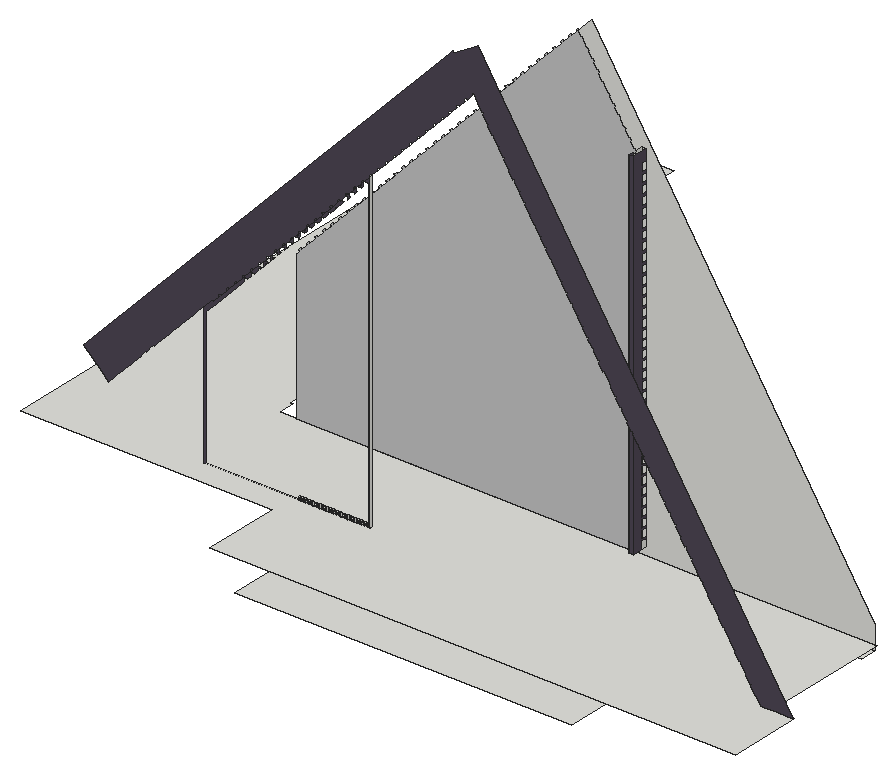
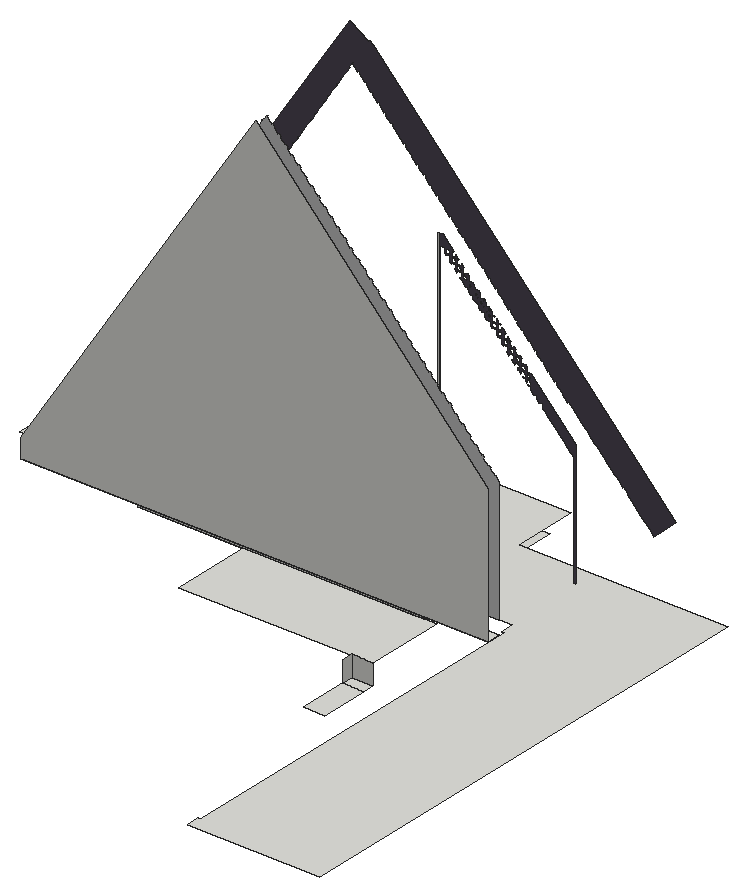
# SketchUp Ruby script. Lengths in inches.
U = 1.inch
M = Sketchup.active_model
def pt(a) = Geom::Point3d.new(a.map { |v| v * U })
def face(e, loops, mat)
  f = e.add_face(loops[0].map { |a| pt(a) })
  loops[1..].each { |l| e.add_face(l.map { |a| pt(a) }).erase! }
  f.material = f.back_material = mat if mat
  f
end
# faces: each face lists its corners as indices into pts; further lists are holes
def faces(e, pts, list, mat = nil) = list.each { |f| face(e, (f[0].is_a?(Array) ? f : [f]).map { |l| l.map { |i| pts[i] } }, mat) }
# xy, xz, yz: faces in a plane at the given z, y or x. An outline is a flat list of corners, or four numbers for a rectangle; further outlines are holes
def ring(l) = l.size == 4 ? [[l[0], l[1]], [l[2], l[1]], [l[2], l[3]], [l[0], l[3]]] : l.each_slice(2).to_a
def flat(e, list, mat, &to3) = list.each { |f| face(e, (f[0].is_a?(Array) ? f : [f]).map { |l| ring(l).map { |u, v| to3.(u, v) } }, mat) }
def xy(e, z, list, mat = nil) = flat(e, list, mat) { |x, y| [x, y, z] }
def xz(e, y, list, mat = nil) = flat(e, list, mat) { |x, z| [x, y, z] }
def yz(e, x, list, mat = nil) = flat(e, list, mat) { |y, z| [x, y, z] }
def lines(e, pts, list) = list.each { |a, b| e.add_line(pt(pts[a]), pt(pts[b])) }
# prism: a flat outline (further loops are holes) pulled along v
def prism(e, loops, v, mat = nil)
  f = face(e, loops, mat); d = Geom::Vector3d.new(v.map { |x| x * U })
  f.pushpull(f.normal.samedirection?(d) ? d.length : -d.length)
end
def box(e, o, s, mat = nil) = prism(e, [[o, [o[0] + s[0], o[1], o[2]], [o[0] + s[0], o[1] + s[1], o[2]], [o[0], o[1] + s[1], o[2]]]], [0, 0, s[2]], mat)
def at(x, y, z, deg = 0) = Geom::Transformation.translation(pt([x, y, z])) * Geom::Transformation.rotation(ORIGIN, Z_AXIS, deg.degrees)
def axes(o, x, y, z) = Geom::Transformation.new([*x, 0, *y, 0, *z, 0, *pt(o).to_a, 1])
def part(name) = M.definitions.add(name)
# library, detail: a bought-in or finely detailed component or shape, given as its bounding box
def library(name, o, s) = part(name).tap { |d| box(d.entities, o, s) }
def detail(e, o, s) = box(e.add_group.entities, o, s)
def put(e, d, t, mat = nil) = e.add_instance(d, t).tap { |i| i.material = mat if mat }
def group(e, t, mat = nil) = e.add_group.tap { |g| g.transformation = t; g.material = mat if mat }.entities
root = M.entities
M.materials.add("[Color M02]").color = [198, 198, 198]
M.materials.add("[Color M06]").color = [79, 71, 84]
c1 = library("A$C06767DEF\#1",[-8.3,1.21,0],[7.09,7.09,5.51])
xy(root,240.465,[[468.015,561.375,478.78,567.012],[468.015,567.012,478.78,591.8125]])
xy(root,250.875,[[[478.547,437.0625,478.547,509.6875,565.03,509.6875,565.03,521.5625,618.43,521.5625,618.43,437.0625],[584.462,456.394,586.015,456.598,587.462,457.198,588.705,458.151,589.659,459.394,590.258,460.841,590.462,462.394,590.258,463.947,589.659,465.394,588.705,466.637,587.462,467.59,586.015,468.189,584.462,468.394,582.91,468.189,581.462,467.59,580.22,466.637,579.266,465.394,578.667,463.947,578.462,462.394,578.667,460.841,579.266,459.394,580.22,458.151,581.462,457.198,582.91,456.598],[521.385,459.394,522.9375,459.598,524.385,460.198,525.627,461.151,526.581,462.394,527.18,463.841,527.385,465.394,527.18,466.947,526.581,468.394,525.627,469.637,524.385,470.59,522.9375,471.189,521.385,471.394,519.832,471.189,518.385,470.59,517.142,469.637,516.188,468.394,515.589,466.947,515.385,465.394,515.589,463.841,516.188,462.394,517.142,461.151,518.385,460.198,519.832,459.598]]])
xy(root,251.0625,[[478.547,509.6875,565.03,521.5625],[468.015,521.5625,468.015,561.375,478.78,561.375,478.78,562.325,565.03,562.325,565.03,521.5625]])
xy(root,252.25,[[584.462,456.394,582.91,456.598,581.462,457.198,580.22,458.151,579.266,459.394,578.667,460.841,578.462,462.394,578.667,463.947,579.266,465.394,580.22,466.637,581.462,467.59,582.91,468.189,584.462,468.394,586.015,468.189,587.462,467.59,588.705,466.637,589.659,465.394,590.258,463.947,590.462,462.394,590.258,460.841,589.659,459.394,588.705,458.151,587.462,457.198,586.015,456.598]])
xy(root,252.375,[[521.385,459.394,519.832,459.598,518.385,460.198,517.142,461.151,516.188,462.394,515.589,463.841,515.385,465.394,515.589,466.947,516.188,468.394,517.142,469.637,518.385,470.59,519.832,471.189,521.385,471.394,522.9375,471.189,524.385,470.59,525.627,469.637,526.581,468.394,527.18,466.947,527.385,465.394,527.18,463.841,526.581,462.394,525.627,461.151,524.385,460.198,522.9375,459.598]])
xy(root,257.0625,[[436.501,521.5625,671.459,528.483]])
xy(root,259.684,[[470.59,480.141,472.903,480.766],[473.502,480.141,475.815,480.766],[476.415,480.141,478.727,480.766],[479.327,480.141,481.639,480.766],[482.239,480.141,484.551,480.766],
  [485.151,480.141,487.463,480.766],[488.0625,480.141,490.375,480.766],[490.975,480.141,493.287,480.766],[493.887,480.141,496.199,480.766],[496.799,480.141,499.111,480.766]])
xy(root,261.996,[[470.59,480.141,472.903,480.766],[473.502,480.141,475.815,480.766],[476.415,480.141,478.727,480.766],[479.327,480.141,481.639,480.766],[482.239,480.141,484.551,480.766],
  [485.151,480.141,487.463,480.766],[488.0625,480.141,490.375,480.766],[490.975,480.141,493.287,480.766],[493.887,480.141,496.199,480.766],[496.799,480.141,499.111,480.766]])
xy(root,262.728,[[470.619,480.141,472.932,480.766],[473.531,480.141,475.844,480.766],[476.444,480.141,478.756,480.766],[479.356,480.141,481.668,480.766],[482.268,480.141,484.58,480.766],
  [485.18,480.141,487.492,480.766],[488.092,480.141,490.404,480.766],[491.004,480.141,493.316,480.766],[493.916,480.141,496.228,480.766],[496.828,480.141,499.14,480.766]])
xy(root,263.889,[[[468.015,437.0625,686.843,437.0625,686.843,467.1875,677.53,467.1875,677.53,521.5625,610.899,521.5625,610.899,519.6875,609.024,519.6875,609.024,521.5625,578.055,521.5625,578.055,519.6875,576.305,519.6875,576.305,521.5625,429.581,521.5625,429.581,528.483,428.001,528.483,428.001,719.591,429.581,719.591,429.581,726.125,363.018,726.125,363.018,469.875,468.015,469.875],[430.975,480.141,500.287,480.766]],[576.305,519.6875,578.055,521.5625],[576.305,521.5625,578.055,526.125]])
xy(root,265.041,[[470.619,480.141,472.932,480.766],[473.531,480.141,475.844,480.766],[476.444,480.141,478.756,480.766],[479.356,480.141,481.668,480.766],[482.268,480.141,484.58,480.766],
  [485.18,480.141,487.492,480.766],[488.092,480.141,490.404,480.766],[491.004,480.141,493.316,480.766],[493.916,480.141,496.228,480.766],[496.828,480.141,499.14,480.766]])
xz(root,467.1875,[[677.53,257.0625,677.53,263.889,686.294,263.889,562.868,456.408,555.191,468.382,549.93,465.009,545.536,462.192,544.977,462.718,543.649,461.307,391.444,299.61,398.981,292.515,402.121,289.56,404.542,292.132,405.42,293.064,407.841,295.636,408.718,296.568,411.139,299.14,412.017,300.072,414.438,302.644,415.315,303.577,415.088,303.791,417.509,306.363,417.737,306.149,418.614,307.081,418.386,307.295,420.808,309.867,421.035,309.653,421.912,310.585,424.334,313.157,425.211,314.089,427.632,316.661,428.51,317.594,430.931,320.166,431.808,321.098,434.229,323.67,435.107,324.602,437.528,327.174,438.405,328.106,440.826,330.678,441.704,331.611,444.125,334.183,445.002,335.115,445.457,334.686,447.878,337.259,447.423,337.687,448.301,338.619,448.756,338.191,451.177,340.763,450.722,341.191,451.599,342.123,452.054,341.695,454.476,344.267,454.02,344.695,454.898,345.628,455.353,345.199,457.774,347.771,457.319,348.2,458.196,349.132,458.652,348.703,461.073,351.276,460.618,351.704,461.495,352.636,461.95,352.208,464.371,354.78,463.916,355.208,464.794,356.14,465.249,355.712,467.67,358.284,467.215,358.712,468.092,359.645,468.547,359.216,470.968,361.788,470.513,362.217,471.391,363.149,471.846,362.72,474.267,365.293,473.812,365.721,474.689,366.653,475.144,366.225,477.565,368.797,477.11,369.225,477.988,370.157,478.443,369.729,480.864,372.301,480.409,372.729,481.286,373.662,481.741,373.233,484.162,375.805,483.707,376.234,484.585,377.166,485.04,376.737,487.461,379.31,487.006,379.738,487.883,380.67,488.338,380.242,490.76,382.814,490.304,383.242,491.182,384.174,491.637,383.746,494.058,386.318,493.603,386.746,494.48,387.679,494.935,387.25,497.357,389.822,496.901,390.251,497.779,391.183,498.234,390.754,500.655,393.327,500.2,393.755,501.077,394.687,501.533,394.259,503.954,396.831,503.499,397.259,504.376,398.191,504.831,397.763,507.252,400.335,506.797,400.763,507.675,401.696,508.13,401.267,510.551,403.839,510.096,404.268,510.973,405.2,511.428,404.771,513.849,407.344,513.394,407.772,514.272,408.704,514.727,408.276,517.148,410.848,516.693,411.276,517.57,412.208,518.025,411.78,520.446,414.352,519.991,414.78,520.869,415.713,521.324,415.284,523.745,417.856,523.29,418.285,524.167,419.217,524.622,418.788,527.043,421.361,526.588,421.789,527.466,422.721,527.921,422.293,530.342,424.865,529.887,425.293,530.764,426.225,531.219,425.797,533.641,428.369,533.185,428.797,534.063,429.73,534.518,429.301,536.939,431.873,536.484,432.302,537.361,433.234,537.817,432.805,540.238,435.378,539.783,435.806,540.66,436.738,541.115,436.31,543.536,438.882,543.081,439.31,543.959,440.242,544.414,439.814,546.835,442.386,546.38,442.814,547.257,443.747,547.712,443.318,550.133,445.89,549.678,446.319,550.556,447.251,551.011,446.822,553.432,449.395,552.977,449.823,553.246,450.109,553.187,450.201,553.555,450.4375,555.124,447.99,555.622,447.213,555.254,446.977,556.948,444.334,557.317,444.57,557.815,443.793,557.447,443.557,559.141,440.914,559.509,441.15,560.008,440.373,559.639,440.137,561.334,437.494,561.702,437.73,562.2,436.953,561.832,436.717,563.526,434.074,563.895,434.31,564.393,433.533,564.024,433.297,565.719,430.654,566.087,430.89,566.585,430.113,566.217,429.877,567.911,427.234,568.28,427.47,568.778,426.693,568.41,426.457,570.104,423.814,570.472,424.05,570.97,423.273,570.602,423.037,572.297,420.394,572.665,420.63,573.163,419.853,572.795,419.617,574.489,416.974,574.858,417.21,575.356,416.433,574.987,416.197,576.682,413.554,577.05,413.79,577.548,413.013,577.18,412.777,578.874,410.134,579.243,410.37,579.741,409.593,579.373,409.357,581.067,406.714,581.435,406.95,581.933,406.173,581.565,405.937,583.26,403.294,583.628,403.53,584.126,402.753,583.758,402.517,585.452,399.874,585.821,400.11,586.319,399.333,585.95,399.097,587.645,396.454,588.013,396.69,588.511,395.913,588.143,395.677,589.837,393.034,590.206,393.27,590.704,392.493,590.336,392.257,592.03,389.614,592.398,389.85,592.896,389.073,592.528,388.837,594.223,386.194,594.591,386.43,595.089,385.653,594.721,385.417,596.415,382.774,596.784,383.01,597.282,382.233,596.913,381.997,598.608,379.354,598.976,379.59,599.474,378.813,599.106,378.577,600.8,375.934,601.169,376.17,601.667,375.393,601.299,375.157,602.993,372.514,603.361,372.75,603.859,371.973,603.491,371.737,605.186,369.094,605.554,369.33,606.187,368.343,605.819,368.106,607.513,365.464,607.881,365.7,608.515,364.712,610.209,362.069,610.842,361.082,610.474,360.846,612.168,358.203,612.536,358.439,613.17,357.451,612.801,357.215,614.496,354.572,614.864,354.808,615.497,353.821,615.129,353.585,616.823,350.942,617.192,351.178,617.825,350.19,617.456,349.954,619.151,347.311,619.519,347.547,620.152,346.56,619.784,346.324,621.478,343.681,621.847,343.917,622.48,342.929,622.111,342.693,623.806,340.05,624.174,340.286,624.706,339.457,624.338,339.221,626.032,336.578,626.4,336.814,626.932,335.984,626.564,335.748,628.258,333.105,628.627,333.341,629.159,332.512,628.79,332.275,630.485,329.632,630.853,329.869,631.385,329.039,631.017,328.803,632.711,326.16,633.079,326.396,633.611,325.566,633.243,325.33,634.9375,322.687,635.306,322.923,635.838,322.094,635.469,321.858,637.164,319.215,637.532,319.451,638.064,318.621,637.696,318.385,639.39,315.742,639.758,315.978,640.29,315.148,639.922,314.912,641.616,312.269,641.985,312.505,642.517,311.676,642.148,311.44,643.843,308.797,644.211,309.033,644.743,308.203,644.375,307.967,646.069,305.324,646.4375,305.56,646.969,304.731,646.601,304.494,648.295,301.851,648.664,302.088,649.196,301.258,648.933,301.089,650.627,298.446,650.89,298.615,651.422,297.785,651.159,297.617,652.853,294.974,653.116,295.142,653.648,294.313,653.385,294.144,655.08,291.501,655.343,291.67,655.875,290.84,655.612,290.671,657.306,288.028,657.569,288.197,658.101,287.367,657.838,287.199,659.532,284.556,659.795,284.724,660.327,283.895,660.064,283.726,661.759,281.083,662.022,281.252,662.554,280.422,662.291,280.254,663.985,277.611,664.248,277.779,664.78,276.95,664.517,276.781,666.211,274.138,666.474,274.307,667.006,273.477,666.743,273.308,668.4375,270.665,668.701,270.834,669.233,270.004,668.97,269.836,670.664,267.193,670.927,267.361,671.459,266.532,671.196,266.363,672.89,263.72,673.153,263.889]],"[Color M06]")
xz(root,480.141,[[499.711,258.951,500.287,263.889],[470.619,262.728,472.932,263.889],[473.531,262.728,475.844,263.889],[476.444,262.728,478.756,263.889],[479.356,262.728,481.668,263.889],
  [482.268,262.728,484.58,263.889],[485.18,262.728,487.492,263.889],[488.092,262.728,490.404,263.889],[491.004,262.728,493.316,263.889],[493.916,262.728,496.228,263.889],
  [496.828,262.728,499.14,263.889]])
xz(root,480.141,[[[430.975,263.889,432.113,263.889,432.113,320.238,433.198,321.395,433.729,321.962,436.11,324.502,436.11,324.774,436.365,324.774,444.846,333.822,446.91,336.024,447.758,336.929,447.758,338.837,449.546,338.837,450.67,340.036,450.67,341.649,452.182,341.649,453.582,343.143,453.582,344.462,454.818,344.462,455.287,344.962,453.582,344.962,453.582,345.956,454.818,347.274,455.895,347.274,455.895,345.61,456.494,346.25,456.494,347.274,457.454,347.274,457.923,347.774,456.494,347.774,456.494,349.0625,457.454,350.087,458.807,350.087,458.807,348.717,459.406,349.357,459.406,350.087,460.09,350.087,460.559,350.587,459.406,350.587,459.406,352.169,460.09,352.899,461.719,352.899,461.719,351.824,462.318,352.464,462.318,352.899,462.726,352.899,463.195,353.399,462.318,353.399,462.318,355.276,462.726,355.712,464.631,355.712,464.631,354.931,465.23,355.571,465.23,355.712,465.362,355.712,465.831,356.212,465.23,356.212,465.23,358.524,467.543,358.524,467.543,358.038,468.467,359.024,468.142,359.024,468.142,361.337,470.455,361.337,470.455,361.145,471.103,361.837,471.054,361.837,471.054,364.149,473.271,364.149,473.966,364.891,473.966,366.962,475.907,366.962,476.878,367.998,476.878,369.774,478.543,369.774,479.012,370.274,479.191,370.466,479.79,371.105,479.79,372.587,481.179,372.587,481.648,373.087,482.103,373.573,482.703,374.212,482.703,375.399,483.815,375.399,484.225,375.837,485.015,376.679,485.615,377.319,485.615,378.149,486.393,378.149,486.803,378.587,487.927,379.786,488.527,380.426,488.527,380.899,488.97,380.899,489.38,381.337,488.527,381.337,488.527,383.649,490.839,383.649,490.839,382.893,491.439,383.533,491.439,383.649,491.548,383.649,491.637,383.746,491.958,384.087,491.439,384.087,491.439,386.399,493.751,386.399,493.751,386,494.535,386.837,494.351,386.837,494.351,389.149,496.663,389.149,496.663,389.107,497.263,389.747,497.263,391.899,499.28,391.899,499.711,392.359,499.711,263.889,500.287,263.889,500.287,397.749,498.037,397.749,492.531,391.899,493.751,391.899,493.751,389.587,491.439,389.587,491.439,390.739,490.839,390.102,490.839,389.587,490.354,389.587,489.942,389.149,490.839,389.149,490.839,386.837,488.527,386.837,488.527,387.645,487.927,387.008,487.927,386.837,487.765,386.837,487.354,386.399,487.927,386.399,487.927,384.087,485.615,384.087,485.615,384.552,484.765,383.649,485.015,383.649,485.015,381.337,482.703,381.337,482.703,381.458,482.103,380.821,482.103,378.587,480,378.587,479.191,377.727,479.191,375.837,477.411,375.837,476.999,375.399,478.543,375.399,476.878,373.623,476.878,375.271,476.279,374.634,476.279,373.087,474.823,373.087,474.352,372.587,475.907,372.587,473.966,370.516,473.966,372.177,473.367,371.54,473.367,370.274,472.175,370.274,471.705,369.774,473.367,369.774,473.367,367.462,471.054,367.462,471.054,369.083,470.455,368.447,470.455,367.462,469.528,367.462,469.057,366.962,470.455,366.962,470.455,364.649,468.142,364.649,468.142,365.99,467.543,365.353,467.543,364.649,466.88,364.649,466.41,364.149,467.543,364.149,467.543,361.837,465.23,361.837,465.23,362.896,464.631,362.259,464.631,361.837,464.233,361.837,463.762,361.337,464.631,361.337,464.631,360.556,463.195,359.024,462.318,359.024,462.318,359.803,461.719,359.166,461.719,359.024,461.586,359.024,461.115,358.524,461.719,358.524,461.719,357.449,460.559,356.212,459.406,356.212,459.406,356.709,458.468,355.712,458.807,355.712,458.807,353.399,456.494,353.399,456.494,353.615,455.82,352.899,455.895,352.899,455.895,350.587,453.643,350.587,430.975,326.504],[468.142,361.837,470.455,364.149],[471.054,364.649,473.367,366.962],[494.351,389.587,496.663,391.899],[491.439,386.837,491.439,387.983,492.536,389.149,493.751,389.149,493.751,386.837],[465.23,359.024,465.23,360.14,466.356,361.337,467.543,361.337,467.543,359.024],[456.494,350.587,456.494,351.875,457.454,352.899,458.807,352.899,458.807,351.53,457.923,350.587],[459.406,353.399,459.406,354.982,460.09,355.712,461.719,355.712,461.719,354.637,460.559,353.399],[453.582,347.774,453.582,348.768,454.818,350.087,455.895,350.087,455.895,348.423,455.287,347.774],[488.527,384.087,488.527,384.89,489.948,386.399,490.839,386.399,490.839,384.087],[462.318,356.212,462.318,358.089,462.726,358.524,464.631,358.524,464.631,357.744,463.195,356.212],[485.615,381.337,485.615,381.796,487.359,383.649,487.927,383.649,487.927,381.337],[482.703,378.587,482.703,378.702,484.77,380.899,485.015,380.899,485.015,378.587],[480.005,375.837,482.103,378.065,482.103,375.837],[473.966,367.704,473.966,369.774,475.907,369.774],[477.417,373.087,479.191,374.972,479.191,373.087],[476.878,370.811,476.878,372.587,478.543,372.587],[474.769,370.274,476.279,371.878,476.279,370.274],[479.79,373.918,479.79,375.399,481.179,375.399],[479.79,376.668,479.79,378.149,481.179,378.149],[482.703,376.962,482.703,378.149,483.815,378.149],[482.703,379.712,482.703,380.899,483.815,380.899],[485.615,380.069,485.615,380.899,486.393,380.899],[485.615,382.819,485.615,383.649,486.393,383.649],[464.18,359.024,464.631,359.504,464.631,359.024],[488.527,385.926,488.527,386.399,488.97,386.399],[461.532,356.212,461.719,356.41,461.719,356.212],[465.23,361.196,465.23,361.337,465.362,361.337],[491.439,389.033,491.439,389.149,491.548,389.149]]],"[Color M06]")
xz(root,480.766,[[470.619,262.728,472.932,263.889],[473.531,262.728,475.844,263.889],[476.444,262.728,478.756,263.889],[479.356,262.728,481.668,263.889],[482.268,262.728,484.58,263.889],
  [485.18,262.728,487.492,263.889],[488.092,262.728,490.404,263.889],[491.004,262.728,493.316,263.889],[493.916,262.728,496.228,263.889],[496.828,262.728,499.14,263.889]])
xz(root,509.6875,[[478.547,250.875,565.03,251.0625]])
xz(root,519.6875,[[576.305,263.889,578.055,412.223]],"[Color M06]")
xz(root,521.5625,[[473.735,246.25,478.547,251.0625],[473.735,251.0625,478.547,257.0625],[478.547,251.0625,618.43,257.0625],[468.015,257.0625,473.735,258.951],[473.735,257.0625,478.547,258.951],
  [478.547,257.0625,618.43,258.951],[468.015,258.951,473.735,263.889],[473.735,258.951,478.547,263.889],[478.547,258.951,618.43,263.889]])
xz(root,521.5625,[[436.501,263.889,576.305,263.889,576.305,412.223,577.535,412.223,577.237,412.689,577.605,412.925,577.05,413.79,576.682,413.554,575.494,415.407,575.044,416.109,575.412,416.345,574.858,417.21,574.489,416.974,573.301,418.827,572.852,419.529,573.22,419.765,572.665,420.63,572.297,420.394,571.109,422.247,570.659,422.949,571.027,423.185,570.472,424.05,570.104,423.814,568.916,425.667,568.466,426.369,568.835,426.605,568.28,427.47,567.911,427.234,566.724,429.087,566.274,429.789,566.642,430.025,566.087,430.89,565.719,430.654,564.531,432.507,564.081,433.209,564.449,433.445,563.895,434.31,563.526,434.074,562.338,435.927,561.889,436.629,562.257,436.865,561.702,437.73,561.334,437.494,560.146,439.347,559.696,440.049,560.064,440.285,559.509,441.15,559.141,440.914,557.953,442.767,557.503,443.469,557.872,443.705,557.317,444.57,556.948,444.334,555.761,446.187,555.311,446.889,555.679,447.125,555.124,447.99,554.756,447.754,553.568,449.607,553.246,450.109,552.977,449.823,553.432,449.395,551.011,446.822,550.556,447.251,549.678,446.319,550.133,445.89,547.712,443.318,547.257,443.747,546.38,442.814,546.835,442.386,544.414,439.814,543.959,440.242,543.081,439.31,543.536,438.882,541.115,436.31,540.66,436.738,539.783,435.806,540.238,435.378,537.817,432.805,537.361,433.234,536.484,432.302,536.939,431.873,534.518,429.301,534.063,429.73,533.185,428.797,533.641,428.369,531.219,425.797,530.764,426.225,529.887,425.293,530.342,424.865,527.921,422.293,527.466,422.721,526.588,421.789,527.043,421.361,524.622,418.788,524.167,419.217,523.29,418.285,523.745,417.856,521.324,415.284,520.869,415.713,519.991,414.78,520.446,414.352,518.025,411.78,517.57,412.208,516.693,411.276,517.148,410.848,514.727,408.276,514.272,408.704,513.394,407.772,513.849,407.344,511.428,404.771,510.973,405.2,510.096,404.268,510.551,403.839,508.13,401.267,507.675,401.696,506.797,400.763,507.252,400.335,504.831,397.763,504.376,398.191,503.499,397.259,503.954,396.831,501.533,394.259,501.077,394.687,500.2,393.755,500.655,393.327,498.234,390.754,497.779,391.183,496.901,390.251,497.357,389.822,494.935,387.25,494.48,387.679,493.603,386.746,494.058,386.318,491.637,383.746,491.182,384.174,490.304,383.242,490.76,382.814,488.338,380.242,487.883,380.67,487.006,379.738,487.461,379.31,485.04,376.737,484.585,377.166,483.707,376.234,484.162,375.805,481.741,373.233,481.286,373.662,480.409,372.729,480.864,372.301,478.443,369.729,477.988,370.157,477.11,369.225,477.565,368.797,475.144,366.225,474.689,366.653,473.812,365.721,474.267,365.293,471.846,362.72,471.391,363.149,470.513,362.217,470.968,361.788,468.547,359.216,468.092,359.645,467.215,358.712,467.67,358.284,465.249,355.712,464.794,356.14,463.916,355.208,464.371,354.78,461.95,352.208,461.495,352.636,460.618,351.704,461.073,351.276,458.652,348.703,458.196,349.132,457.319,348.2,457.774,347.771,455.353,345.199,454.898,345.628,454.02,344.695,454.476,344.267,452.054,341.695,451.599,342.123,450.722,341.191,451.177,340.763,450.577,340.125,450.173,339.697,448.756,338.191,448.301,338.619,447.423,337.687,447.878,337.259,445.457,334.686,445.002,335.115,444.125,334.183,444.58,333.754,442.159,331.182,441.704,331.611,440.826,330.678,441.281,330.25,438.86,327.678,438.405,328.106,437.528,327.174,437.983,326.746,436.956,325.655,436.501,325.171]],"[Color M02]")
xz(root,526.125,[[576.305,263.889,578.055,412.223]])
xz(root,528.483,[[436.501,257.0625,436.501,326.083,553.555,450.4375,671.459,266.532,671.459,257.0625]])
xz(root,561.375,[[468.015,240.465,478.78,251.0625]])
yz(root,472.903,[[480.141,259.684,480.766,261.996]])
yz(root,472.932,[[480.141,262.728,480.766,265.041]])
yz(root,473.502,[[480.141,259.684,480.766,261.996]])
yz(root,473.531,[[480.141,262.728,480.766,265.041]])
yz(root,475.815,[[480.141,259.684,480.766,261.996]])
yz(root,475.844,[[480.141,262.728,480.766,265.041]])
yz(root,476.415,[[480.141,259.684,480.766,261.996]])
yz(root,476.444,[[480.141,262.728,480.766,265.041]])
yz(root,478.547,[[509.6875,246.25,521.5625,251.0625]])
yz(root,478.727,[[480.141,259.684,480.766,261.996]])
yz(root,478.756,[[480.141,262.728,480.766,265.041]])
yz(root,478.78,[[561.375,240.465,567.012,251.0625]])
yz(root,479.327,[[480.141,259.684,480.766,261.996]])
yz(root,479.356,[[480.141,262.728,480.766,265.041]])
yz(root,481.639,[[480.141,259.684,480.766,261.996]])
yz(root,481.668,[[480.141,262.728,480.766,265.041]])
yz(root,482.239,[[480.141,259.684,480.766,261.996]])
yz(root,482.268,[[480.141,262.728,480.766,265.041]])
yz(root,484.551,[[480.141,259.684,480.766,261.996]])
yz(root,484.58,[[480.141,262.728,480.766,265.041]])
yz(root,485.151,[[480.141,259.684,480.766,261.996]])
yz(root,485.18,[[480.141,262.728,480.766,265.041]])
yz(root,487.463,[[480.141,259.684,480.766,261.996]])
yz(root,487.492,[[480.141,262.728,480.766,265.041]])
yz(root,488.0625,[[480.141,259.684,480.766,261.996]])
yz(root,488.092,[[480.141,262.728,480.766,265.041]])
yz(root,490.375,[[480.141,259.684,480.766,261.996]])
yz(root,490.404,[[480.141,262.728,480.766,265.041]])
yz(root,490.975,[[480.141,259.684,480.766,261.996]])
yz(root,491.004,[[480.141,262.728,480.766,265.041]])
yz(root,493.287,[[480.141,259.684,480.766,261.996]])
yz(root,493.316,[[480.141,262.728,480.766,265.041]])
yz(root,493.887,[[480.141,259.684,480.766,261.996]])
yz(root,493.916,[[480.141,262.728,480.766,265.041]])
yz(root,496.199,[[480.141,259.684,480.766,261.996]])
yz(root,496.228,[[480.141,262.728,480.766,265.041]])
yz(root,496.799,[[480.141,259.684,480.766,261.996]])
yz(root,496.828,[[480.141,262.728,480.766,265.041]])
yz(root,499.111,[[480.141,259.684,480.766,261.996]])
yz(root,499.14,[[480.141,262.728,480.766,265.041]])
yz(root,500.287,[[480.141,258.951,480.766,263.889],[480.141,263.889,480.766,397.749]])
yz(root,565.03,[[509.6875,250.875,521.5625,251.0625]])
yz(root,576.305,[[521.5625,263.889,526.125,412.223]])
yz(root,576.305,[[519.6875,263.889,521.5625,412.223]],"[Color M06]")
yz(root,578.055,[[523.75,263.889,526.125,267.016]])
yz(root,578.055,[[519.6875,263.889,523.75,263.889,523.75,267.016,526.125,267.016,526.125,267.826,523.75,267.826,523.75,270.953,526.125,270.953,526.125,271.764,523.75,271.764,523.75,274.891,526.125,274.891,526.125,275.701,523.75,275.701,523.75,278.828,526.125,278.828,526.125,279.639,523.75,279.639,523.75,282.766,526.125,282.766,526.125,283.576,523.75,283.576,523.75,286.703,526.125,286.703,526.125,287.514,523.75,287.514,523.75,290.641,526.125,290.641,526.125,291.451,523.75,291.451,523.75,294.578,526.125,294.578,526.125,295.389,523.75,295.389,523.75,298.516,526.125,298.516,526.125,299.326,523.75,299.326,523.75,302.453,526.125,302.453,526.125,303.264,523.75,303.264,523.75,306.391,526.125,306.391,526.125,307.201,523.75,307.201,523.75,310.328,526.125,310.328,526.125,311.139,523.75,311.139,523.75,314.266,526.125,314.266,526.125,315.076,524.25,315.076,524.25,318.203,526.125,318.203,526.125,319.014,524.25,319.014,524.25,322.141,526.125,322.141,526.125,322.889,524.25,322.889,524.25,326.016,526.125,326.016,526.125,326.764,524.25,326.764,524.25,329.891,526.125,329.891,526.125,330.639,524.25,330.639,524.25,333.766,526.125,333.766,526.125,334.514,524.25,334.514,524.25,337.641,526.125,337.641,526.125,338.389,524.25,338.389,524.25,341.516,526.125,341.516,526.125,341.933,524.25,341.933,524.25,345.06,526.125,345.06,526.125,345.995,524.25,345.995,524.25,349.122,526.125,349.122,526.125,350.058,524.25,350.058,524.25,353.185,526.125,353.185,526.125,354.12,524.25,354.12,524.25,357.247,526.125,357.247,526.125,358.058,524.25,358.058,524.25,361.185,526.125,361.185,526.125,361.995,524.25,361.995,524.25,365.122,526.125,365.122,526.125,366.245,524.25,366.245,524.25,369.372,526.125,369.372,526.125,370.495,524.25,370.495,524.25,373.622,526.125,373.622,526.125,374.745,524.25,374.745,524.25,377.872,526.125,377.872,526.125,378.995,524.25,378.995,524.25,382.122,526.125,382.122,526.125,383.245,524.25,383.245,524.25,386.372,526.125,386.372,526.125,387.495,524.25,387.495,524.25,390.622,526.125,390.622,526.125,391.745,524.25,391.745,524.25,394.872,526.125,394.872,526.125,395.995,524.25,395.995,524.25,399.122,526.125,399.122,526.125,400.245,524.25,400.245,524.25,403.372,526.125,403.372,526.125,404.495,524.25,404.495,524.25,407.622,526.125,407.622,526.125,412.223,519.6875,412.223]],"[Color M06]")
p = [[584.462,456.394,250.875],[582.91,456.598,250.875],[582.91,456.598,252.25],[584.462,456.394,252.25],[586.015,456.598,250.875],[586.015,456.598,252.25],
  [581.462,457.198,250.875],[581.462,457.198,252.25],[580.22,458.151,250.875],[580.22,458.151,252.25],[579.266,459.394,250.875],[579.266,459.394,252.25],
  [521.385,459.394,250.875],[519.832,459.598,250.875],[519.832,459.598,252.375],[521.385,459.394,252.375],[522.9375,459.598,250.875],[522.9375,459.598,252.375],
  [578.667,460.841,250.875],[578.667,460.841,252.25],[518.385,460.198,250.875],[518.385,460.198,252.375],[524.385,460.198,250.875],[524.385,460.198,252.375],
  [517.142,461.151,250.875],[517.142,461.151,252.375],[525.627,461.151,250.875],[525.627,461.151,252.375],[578.462,462.394,250.875],[578.462,462.394,252.25],
  [516.188,462.394,250.875],[516.188,462.394,252.375],[526.581,462.394,250.875],[526.581,462.394,252.375],[515.589,463.841,250.875],[515.589,463.841,252.375],
  [527.18,463.841,250.875],[527.18,463.841,252.375],[578.667,463.947,250.875],[578.667,463.947,252.25],[515.385,465.394,250.875],[515.385,465.394,252.375],
  [527.385,465.394,250.875],[527.385,465.394,252.375],[579.266,465.394,250.875],[579.266,465.394,252.25],[515.589,466.947,250.875],[515.589,466.947,252.375],
  [527.18,466.947,250.875],[527.18,466.947,252.375],[580.22,466.637,250.875],[580.22,466.637,252.25],[581.462,467.59,250.875],[581.462,467.59,252.25],
  [516.188,468.394,250.875],[516.188,468.394,252.375],[526.581,468.394,250.875],[526.581,468.394,252.375],[582.91,468.189,250.875],[582.91,468.189,252.25],
  [584.462,468.394,250.875],[584.462,468.394,252.25],[586.015,468.189,250.875],[586.015,468.189,252.25],[517.142,469.637,250.875],[517.142,469.637,252.375],
  [525.627,469.637,250.875],[525.627,469.637,252.375],[518.385,470.59,250.875],[518.385,470.59,252.375],[524.385,470.59,250.875],[524.385,470.59,252.375],
  [519.832,471.189,250.875],[519.832,471.189,252.375],[522.9375,471.189,250.875],[522.9375,471.189,252.375],[521.385,471.394,250.875],[521.385,471.394,252.375],
  [473.735,521.5625,246.25],[473.735,467.1875,246.25],[473.735,521.5625,251.0625],[473.735,467.1875,251.0625]]
faces(root,p,[[0,1,2,3],[4,0,3,5],[1,6,7,2],[6,8,9,7],[8,10,11,9],[12,13,14,15],[16,12,15,17],[10,18,19,11],
  [13,20,21,14],[22,16,17,23],[20,24,25,21],[26,22,23,27],[18,28,29,19],[24,30,31,25],[32,26,27,33],[30,34,35,31],
  [36,32,33,37],[28,38,39,29],[34,40,41,35],[42,36,37,43],[38,44,45,39],[40,46,47,41],[48,42,43,49],[44,50,51,45],
  [50,52,53,51],[46,54,55,47],[56,48,49,57],[52,58,59,53],[58,60,61,59],[60,62,63,61],[54,64,65,55],[66,56,57,67],
  [64,68,69,65],[70,66,67,71],[68,72,73,69],[74,70,71,75],[72,76,77,73],[76,74,75,77]])
lines(root,p,[[78,79],[80,81]])
put(root,c1,axes([526.99,464.17,249.52],[1.14885,0,0],[0,0.84644,0],[0,0,0.5175]))
put(root,c1,axes([591.05,458.37,248.02],[1.14885,0,0],[0,0.84644,0],[0,0,0.5175]))
